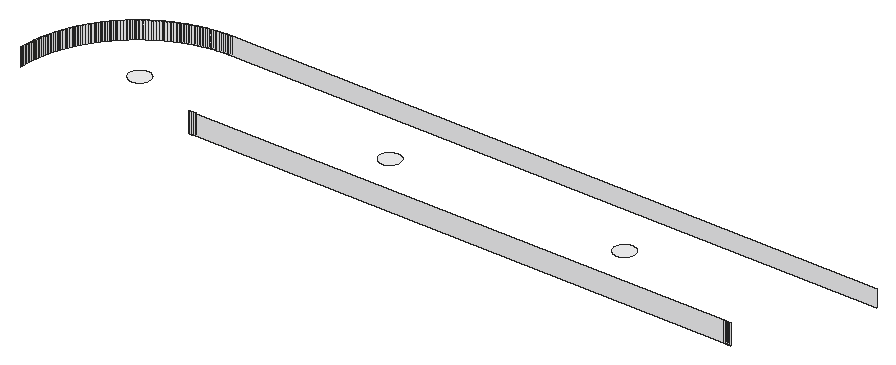
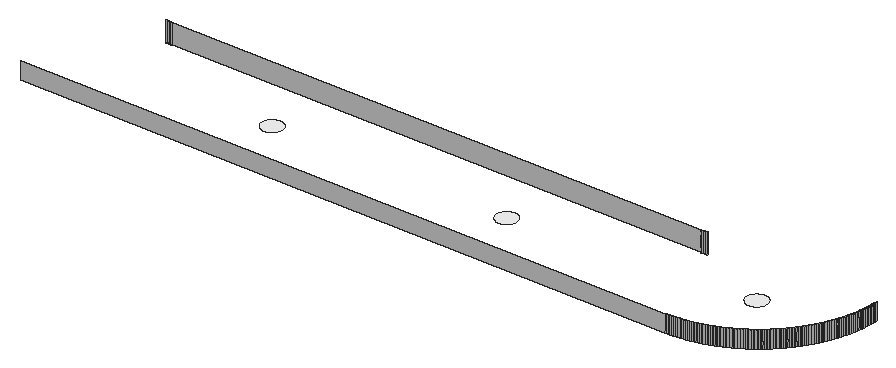
# SketchUp Ruby script. Lengths in inches.
U = 1.inch
M = Sketchup.active_model
def pt(a) = Geom::Point3d.new(a.map { |v| v * U })
def face(e, loops, mat)
  f = e.add_face(loops[0].map { |a| pt(a) })
  loops[1..].each { |l| e.add_face(l.map { |a| pt(a) }).erase! }
  f.material = f.back_material = mat if mat
  f
end
# faces: each face lists its corners as indices into pts; further lists are holes
def faces(e, pts, list, mat = nil) = list.each { |f| face(e, (f[0].is_a?(Array) ? f : [f]).map { |l| l.map { |i| pts[i] } }, mat) }
# xy, xz, yz: faces in a plane at the given z, y or x. An outline is a flat list of corners, or four numbers for a rectangle; further outlines are holes
def ring(l) = l.size == 4 ? [[l[0], l[1]], [l[2], l[1]], [l[2], l[3]], [l[0], l[3]]] : l.each_slice(2).to_a
def flat(e, list, mat, &to3) = list.each { |f| face(e, (f[0].is_a?(Array) ? f : [f]).map { |l| ring(l).map { |u, v| to3.(u, v) } }, mat) }
def xy(e, z, list, mat = nil) = flat(e, list, mat) { |x, y| [x, y, z] }
def xz(e, y, list, mat = nil) = flat(e, list, mat) { |x, z| [x, y, z] }
def yz(e, x, list, mat = nil) = flat(e, list, mat) { |y, z| [x, y, z] }
def lines(e, pts, list) = list.each { |a, b| e.add_line(pt(pts[a]), pt(pts[b])) }
# prism: a flat outline (further loops are holes) pulled along v
def prism(e, loops, v, mat = nil)
  f = face(e, loops, mat); d = Geom::Vector3d.new(v.map { |x| x * U })
  f.pushpull(f.normal.samedirection?(d) ? d.length : -d.length)
end
def box(e, o, s, mat = nil) = prism(e, [[o, [o[0] + s[0], o[1], o[2]], [o[0] + s[0], o[1] + s[1], o[2]], [o[0], o[1] + s[1], o[2]]]], [0, 0, s[2]], mat)
def at(x, y, z, deg = 0) = Geom::Transformation.translation(pt([x, y, z])) * Geom::Transformation.rotation(ORIGIN, Z_AXIS, deg.degrees)
def axes(o, x, y, z) = Geom::Transformation.new([*x, 0, *y, 0, *z, 0, *pt(o).to_a, 1])
def part(name) = M.definitions.add(name)
# library, detail: a bought-in or finely detailed component or shape, given as its bounding box
def library(name, o, s) = part(name).tap { |d| box(d.entities, o, s) }
def detail(e, o, s) = box(e.add_group.entities, o, s)
def put(e, d, t, mat = nil) = e.add_instance(d, t).tap { |i| i.material = mat if mat }
def group(e, t, mat = nil) = e.add_group.tap { |g| g.transformation = t; g.material = mat if mat }.entities
root = M.entities
M.materials.add("[Quartz Light Grey]").color = [251, 251, 252]
xy(root,112.81,[[38.9375,222.06,38.9,222.07,38.8125,222.07,38.77,222.08,38.73,222.08,38.6875,222.09,38.65,222.09,38.625,222.1,38.6,222.1,38.5625,222.11,38.52,222.12,38.4,222.15,38.36,222.17,38.32,222.18,38.28,222.2,38.26,222.2,38.24,222.21,38.21,222.23,38.17,222.24,38.09,222.28,38.06,222.3,38.04,222.3125,38.02,222.32,37.98,222.34,37.95,222.36,37.91,222.39,37.84,222.43,37.81,222.46,37.77,222.48,37.71,222.54,37.68,222.5625,37.65,222.59,37.56,222.68,37.54,222.69,37.53,222.71,37.47,222.77,37.46,222.79,37.45,222.8,37.42,222.84,37.39,222.87,37.38,222.89,37.37,222.9,37.35,222.9375,37.32,222.97,37.3125,222.99,37.3,223.01,37.28,223.05,37.26,223.08,37.22,223.16,37.2,223.19,37.18,223.23,37.17,223.27,37.13,223.35,37.12,223.39,37.1,223.42,37.1,223.44,37.09,223.47,37.08,223.51,37.07,223.54,37.0625,223.57,37.06,223.59,37.05,223.625,37.04,223.67,37.04,223.6875,37.03,223.71,37.03,223.75,37.02,223.79,37.02,223.8125,37.01,223.83,37.01,223.92,37,223.9375,37,224.1875,37.01,224.21,37.01,224.29,37.02,224.3125,37.02,224.33,37.03,224.375,37.03,224.42,37.04,224.4375,37.04,224.46,37.06,224.54,37.0625,224.56,37.07,224.58,37.09,224.66,37.1,224.68,37.1,224.7,37.12,224.74,37.13,224.78,37.17,224.86,37.18,224.89,37.26,225.05,37.28,225.08,37.3,225.12,37.3125,225.13,37.32,225.15,37.35,225.1875,37.37,225.22,37.39,225.26,37.45,225.32,37.46,225.34,37.5,225.38,37.53,225.42,37.65,225.54,37.68,225.5625,37.71,225.59,37.73,225.6,37.74,225.62,37.77,225.64,37.81,225.67,37.82,225.68,37.84,225.69,37.875,225.72,37.91,225.74,37.95,225.76,37.98,225.78,38.04,225.81,38.06,225.83,38.09,225.84,38.21,225.9,38.24,225.91,38.28,225.93,38.32,225.94,38.36,225.96,38.38,225.96,38.4,225.97,38.48,225.99,38.52,226.01,38.5625,226.01,38.6,226.02,38.625,226.03,38.65,226.03,38.6875,226.04,38.73,226.04,38.75,226.05,38.8125,226.05,38.85,226.06,38.9,226.06,38.9375,226.0625,39.0625,226.0625,39.1,226.06,39.15,226.06,39.1875,226.05,39.25,226.05,39.27,226.04,39.3125,226.04,39.35,226.03,39.375,226.03,39.4,226.02,39.4375,226.01,39.48,226.01,39.52,225.99,39.6,225.97,39.62,225.96,39.64,225.96,39.68,225.94,39.72,225.93,39.76,225.91,39.79,225.9,39.91,225.84,39.94,225.83,39.96,225.81,40.02,225.78,40.05,225.76,40.09,225.74,40.125,225.72,40.16,225.69,40.18,225.68,40.19,225.67,40.23,225.64,40.26,225.62,40.27,225.6,40.29,225.59,40.32,225.5625,40.35,225.54,40.47,225.42,40.5,225.38,40.54,225.34,40.55,225.32,40.61,225.26,40.63,225.22,40.65,225.1875,40.68,225.15,40.6875,225.13,40.7,225.12,40.72,225.08,40.74,225.05,40.82,224.89,40.83,224.86,40.87,224.78,40.88,224.74,40.9,224.7,40.9,224.68,40.91,224.66,40.93,224.58,40.9375,224.56,40.94,224.54,40.96,224.46,40.96,224.4375,40.97,224.42,40.97,224.375,40.98,224.33,40.98,224.3125,40.99,224.29,40.99,224.21,41,224.1875,41,223.9375,40.99,223.92,40.99,223.83,40.98,223.8125,40.98,223.79,40.97,223.75,40.97,223.71,40.96,223.6875,40.96,223.67,40.95,223.625,40.94,223.59,40.9375,223.57,40.93,223.54,40.92,223.51,40.91,223.47,40.9,223.44,40.9,223.42,40.88,223.39,40.87,223.35,40.83,223.27,40.82,223.23,40.8,223.19,40.78,223.16,40.74,223.08,40.72,223.05,40.7,223.01,40.6875,222.99,40.68,222.97,40.65,222.9375,40.63,222.9,40.62,222.89,40.61,222.87,40.58,222.84,40.55,222.8,40.54,222.79,40.53,222.77,40.47,222.71,40.46,222.69,40.44,222.68,40.35,222.59,40.32,222.5625,40.29,222.54,40.23,222.48,40.19,222.46,40.16,222.43,40.09,222.39,40.05,222.36,40.02,222.34,39.98,222.32,39.96,222.3125,39.94,222.3,39.91,222.28,39.83,222.24,39.79,222.23,39.76,222.21,39.74,222.2,39.72,222.2,39.68,222.18,39.64,222.17,39.6,222.15,39.48,222.12,39.4375,222.11,39.4,222.1,39.375,222.1,39.35,222.09,39.3125,222.09,39.27,222.08,39.23,222.08,39.1875,222.07,39.1,222.07,39.0625,222.06,39.02,222.0625,38.98,222.0625],[86.98,226.0625,86.85,226.07,86.73,226.08,86.6,226.1,86.48,226.13,86.24,226.21,86.13,226.26,86.02,226.32,85.91,226.39,85.81,226.46,85.71,226.54,85.62,226.62,85.53,226.71,85.45,226.8,85.37,226.9,85.3,227.01,85.18,227.23,85.13,227.35,85.09,227.47,85.03,227.71,85.01,227.83,85,227.96,85,228.08,85.01,228.21,85.02,228.33,85.04,228.46,85.1,228.7,85.15,228.82,85.2,228.93,85.26,229.05,85.32,229.15,85.39,229.26,85.47,229.35,85.56,229.45,85.65,229.54,85.74,229.62,85.84,229.69,86.06,229.83,86.28,229.93,86.52,230.01,86.65,230.03,86.77,230.05,86.9,230.06,87.02,230.0625,87.15,230.06,87.27,230.04,87.4,230.02,87.64,229.96,87.76,229.91,87.87,229.86,88.09,229.74,88.19,229.67,88.29,229.59,88.38,229.51,88.47,229.42,88.63,229.22,88.7,229.12,88.76,229.01,88.82,228.89,88.87,228.78,88.91,228.66,88.97,228.42,88.99,228.29,89,228.17,89,228.04,88.99,227.92,88.98,227.79,88.96,227.67,88.93,227.54,88.9,227.42,88.85,227.31,88.8,227.19,88.68,226.97,88.61,226.87,88.53,226.77,88.35,226.59,88.26,226.51,88.16,226.43,88.05,226.36,87.83,226.24,87.72,226.2,87.6,226.15,87.48,226.12,87.35,226.09,87.23,226.08,87.1,226.07],[134.98,226.0625,134.85,226.07,134.73,226.08,134.6,226.1,134.48,226.13,134.24,226.21,134.13,226.26,134.02,226.32,133.91,226.39,133.81,226.46,133.71,226.54,133.62,226.62,133.53,226.71,133.45,226.8,133.37,226.9,133.3,227.01,133.18,227.23,133.13,227.35,133.09,227.47,133.03,227.71,133.01,227.83,133,227.96,133,228.08,133.01,228.21,133.02,228.33,133.04,228.46,133.1,228.7,133.15,228.82,133.2,228.93,133.26,229.05,133.32,229.15,133.39,229.26,133.47,229.35,133.56,229.45,133.65,229.54,133.74,229.62,133.84,229.69,134.06,229.83,134.28,229.93,134.52,230.01,134.65,230.03,134.77,230.05,134.9,230.06,135.02,230.0625,135.15,230.06,135.27,230.04,135.4,230.02,135.64,229.96,135.76,229.91,135.87,229.86,136.09,229.74,136.19,229.67,136.29,229.59,136.38,229.51,136.47,229.42,136.63,229.22,136.7,229.12,136.76,229.01,136.82,228.89,136.87,228.78,136.91,228.66,136.97,228.42,136.99,228.29,137,228.17,137,228.04,136.99,227.92,136.98,227.79,136.96,227.67,136.93,227.54,136.9,227.42,136.85,227.31,136.8,227.19,136.68,226.97,136.61,226.87,136.53,226.77,136.35,226.59,136.26,226.51,136.16,226.43,136.05,226.36,135.83,226.24,135.72,226.2,135.6,226.15,135.48,226.12,135.35,226.09,135.23,226.08,135.1,226.07]],"[Quartz Light Grey]")
xz(root,216,[[56.6875,111.81,56.84,115.91],[56.84,111.81,57,115.91],[57,111.81,165,115.91],[165,111.81,165.16,115.91],[165.16,111.81,165.3125,115.91]],"[Quartz Light Grey]")
xz(root,239.99,[[44.25,111.81,44.5,115.32]],"[Quartz Light Grey]")
xz(root,240,[[44.75,111.81,45,115.32],[45,111.81,177,115.32]],"[Quartz Light Grey]")
yz(root,21,[[216,111.81,216.25,115.32]],"[Quartz Light Grey]")
yz(root,21.01,[[216.5,111.81,216.75,115.32]],"[Quartz Light Grey]")
p = [[55.59,215.92,111.81],[55.75,215.93,111.81],[55.75,215.93,115.91],[55.59,215.92,115.91],[55.9,215.95,111.81],[55.9,215.95,115.91],
  [56.06,215.96,111.81],[56.06,215.96,115.91],[165.94,215.96,111.81],[166.1,215.95,111.81],[166.1,215.95,115.91],[165.94,215.96,115.91],
  [166.25,215.93,111.81],[166.25,215.93,115.91],[166.41,215.92,111.81],[166.41,215.92,115.91],[56.22,215.97,111.81],[56.22,215.97,115.91],
  [56.37,215.98,111.81],[56.37,215.98,115.91],[56.53,215.99,111.81],[56.53,215.99,115.91],[56.6875,216,111.81],[56.6875,216,115.91],
  [165.3125,216,111.81],[165.47,215.99,111.81],[165.47,215.99,115.91],[165.3125,216,115.91],[165.63,215.98,111.81],[165.63,215.98,115.91],
  [165.78,215.97,111.81],[165.78,215.97,115.91],[21.01,216.5,111.81],[21,216.25,111.81],[21,216.25,115.32],[21.01,216.5,115.32],
  [21.02,217.01,111.81],[21.01,216.75,111.81],[21.01,216.75,115.32],[21.02,217.01,115.32],[21.03,217.26,111.81],[21.03,217.26,115.32],
  [21.05,217.51,111.81],[21.05,217.51,115.32],[21.0625,217.76,111.81],[21.0625,217.76,115.32],[21.08,218.01,111.81],[21.08,218.01,115.32],
  [21.11,218.26,111.81],[21.11,218.26,115.32],[21.13,218.51,111.81],[21.13,218.51,115.32],[21.16,218.76,111.81],[21.16,218.76,115.32],
  [21.1875,219.01,111.81],[21.1875,219.01,115.32],[21.22,219.26,111.81],[21.22,219.26,115.32],[21.26,219.51,111.81],[21.26,219.51,115.32],
  [21.3,219.75,111.81],[21.3,219.75,115.32],[21.34,220,111.81],[21.34,220,115.32],[21.38,220.25,111.81],[21.38,220.25,115.32],
  [21.43,220.5,111.81],[21.43,220.5,115.32],[21.47,220.74,111.81],[21.47,220.74,115.32],[21.52,220.99,111.81],[21.52,220.99,115.32],
  [21.58,221.24,111.81],[21.58,221.24,115.32],[21.63,221.48,111.81],[21.63,221.48,115.32],[21.69,221.72,111.81],[21.69,221.72,115.32],
  [21.75,221.97,111.81],[21.75,221.97,115.32],[21.82,222.21,111.81],[21.82,222.21,115.32],[21.88,222.45,111.81],[21.88,222.45,115.32],
  [21.95,222.7,111.81],[21.95,222.7,115.32],[22.02,222.9375,111.81],[22.02,222.9375,115.32],[22.1,223.18,111.81],[22.1,223.18,115.32],
  [22.17,223.42,111.81],[22.17,223.42,115.32],[22.25,223.66,111.81],[22.25,223.66,115.32],[22.33,223.89,111.81],[22.33,223.89,115.32],
  [22.42,224.13,111.81],[22.42,224.13,115.32],[22.51,224.37,111.81],[22.51,224.37,115.32],[22.59,224.6,111.81],[22.59,224.6,115.32],
  [22.69,224.83,111.81],[22.69,224.83,115.32],[22.78,225.07,111.81],[22.78,225.07,115.32],[22.875,225.3,111.81],[22.875,225.3,115.32],
  [22.97,225.53,111.81],[22.97,225.53,115.32],[23.07,225.76,111.81],[23.07,225.76,115.32],[23.18,225.99,111.81],[23.18,225.99,115.32],
  [23.28,226.22,111.81],[23.28,226.22,115.32],[23.39,226.45,111.81],[23.39,226.45,115.32],[23.5,226.67,111.81],[23.5,226.67,115.32],
  [23.62,226.9,111.81],[23.62,226.9,115.32],[23.73,227.12,111.81],[23.73,227.12,115.32],[23.85,227.34,111.81],[23.85,227.34,115.32],
  [23.97,227.5625,111.81],[23.97,227.5625,115.32],[24.09,227.78,111.81],[24.09,227.78,115.32],[24.22,228,111.81],[24.22,228,115.32],
  [24.34,228.22,111.81],[24.34,228.22,115.32],[24.47,228.43,111.81],[24.47,228.43,115.32],[24.6,228.65,111.81],[24.6,228.65,115.32],
  [24.74,228.86,111.81],[24.74,228.86,115.32],[24.87,229.07,111.81],[24.87,229.07,115.32],[25.01,229.28,111.81],[25.01,229.28,115.32],
  [25.15,229.49,111.81],[25.15,229.49,115.32],[25.29,229.7,111.81],[25.29,229.7,115.32],[25.4375,229.9,111.81],[25.4375,229.9,115.32],
  [25.58,230.11,111.81],[25.58,230.11,115.32],[25.73,230.31,111.81],[25.73,230.31,115.32],[25.88,230.51,111.81],[25.88,230.51,115.32],
  [26.04,230.71,111.81],[26.04,230.71,115.32],[26.19,230.91,111.81],[26.19,230.91,115.32],[26.35,231.1,111.81],[26.35,231.1,115.32],
  [26.51,231.3,111.81],[26.51,231.3,115.32],[26.67,231.49,111.81],[26.67,231.49,115.32],[26.83,231.68,111.81],[26.83,231.68,115.32],
  [27,231.87,111.81],[27,231.87,115.32],[27.16,232.06,111.81],[27.16,232.06,115.32],[27.33,232.25,111.81],[27.33,232.25,115.32],
  [27.5,232.43,111.81],[27.5,232.43,115.32],[27.68,232.61,111.81],[27.68,232.61,115.32],[27.85,232.79,111.81],[27.85,232.79,115.32],
  [28.03,232.97,111.81],[28.03,232.97,115.32],[28.21,233.15,111.81],[28.21,233.15,115.32],[28.39,233.32,111.81],[28.39,233.32,115.32],
  [28.57,233.5,111.81],[28.57,233.5,115.32],[28.75,233.67,111.81],[28.75,233.67,115.32],[28.94,233.84,111.81],[28.94,233.84,115.32],
  [29.13,234,111.81],[29.13,234,115.32],[29.32,234.17,111.81],[29.32,234.17,115.32],[29.51,234.33,111.81],[29.51,234.33,115.32],
  [29.7,234.49,111.81],[29.7,234.49,115.32],[29.9,234.65,111.81],[29.9,234.65,115.32],[30.09,234.81,111.81],[30.09,234.81,115.32],
  [30.29,234.96,111.81],[30.29,234.96,115.32],[30.49,235.12,111.81],[30.49,235.12,115.32],[30.69,235.27,111.81],[30.69,235.27,115.32],
  [30.89,235.42,111.81],[30.89,235.42,115.32],[31.1,235.5625,111.81],[31.1,235.5625,115.32],[31.3,235.71,111.81],[31.3,235.71,115.32],
  [31.51,235.85,111.81],[31.51,235.85,115.32],[31.72,235.99,111.81],[31.72,235.99,115.32],[31.93,236.13,111.81],[31.93,236.13,115.32],
  [32.14,236.26,111.81],[32.14,236.26,115.32],[32.35,236.4,111.81],[32.35,236.4,115.32],[32.57,236.53,111.81],[32.57,236.53,115.32],
  [32.78,236.66,111.81],[32.78,236.66,115.32],[33,236.78,111.81],[33,236.78,115.32],[33.22,236.91,111.81],[33.22,236.91,115.32],
  [33.4375,237.03,111.81],[33.4375,237.03,115.32],[33.66,237.15,111.81],[33.66,237.15,115.32],[33.88,237.27,111.81],[33.88,237.27,115.32],
  [34.1,237.38,111.81],[34.1,237.38,115.32],[34.33,237.5,111.81],[34.33,237.5,115.32],[34.55,237.61,111.81],[34.55,237.61,115.32],
  [34.78,237.72,111.81],[34.78,237.72,115.32],[35.01,237.82,111.81],[35.01,237.82,115.32],[35.24,237.93,111.81],[35.24,237.93,115.32],
  [35.47,238.03,111.81],[35.47,238.03,115.32],[35.7,238.125,111.81],[35.7,238.125,115.32],[35.93,238.22,111.81],[35.93,238.22,115.32],
  [36.17,238.31,111.81],[36.17,238.31,115.32],[36.4,238.41,111.81],[36.4,238.41,115.32],[36.63,238.49,111.81],[36.63,238.49,115.32],
  [36.87,238.58,111.81],[36.87,238.58,115.32],[37.11,238.67,111.81],[37.11,238.67,115.32],[37.34,238.75,111.81],[37.34,238.75,115.32],
  [37.58,238.83,111.81],[37.58,238.83,115.32],[37.82,238.9,111.81],[37.82,238.9,115.32],[38.0625,238.98,111.81],[38.0625,238.98,115.32],
  [38.3,239.05,111.81],[38.3,239.05,115.32],[38.55,239.12,111.81],[38.55,239.12,115.32],[38.79,239.18,111.81],[38.79,239.18,115.32],
  [39.03,239.25,111.81],[39.03,239.25,115.32],[39.28,239.31,111.81],[39.28,239.31,115.32],[39.52,239.37,111.81],[39.52,239.37,115.32],
  [39.76,239.42,111.81],[39.76,239.42,115.32],[40.01,239.48,111.81],[40.01,239.48,115.32],[40.26,239.53,111.81],[40.26,239.53,115.32],
  [40.5,239.57,111.81],[40.5,239.57,115.32],[40.75,239.62,111.81],[40.75,239.62,115.32],[41,239.66,111.81],[41,239.66,115.32],
  [41.25,239.7,111.81],[41.25,239.7,115.32],[41.49,239.74,111.81],[41.49,239.74,115.32],[41.74,239.78,111.81],[41.74,239.78,115.32],
  [41.99,239.8125,111.81],[41.99,239.8125,115.32],[42.24,239.84,111.81],[42.24,239.84,115.32],[42.49,239.87,111.81],[42.49,239.87,115.32],
  [42.74,239.89,111.81],[42.74,239.89,115.32],[42.99,239.92,111.81],[42.99,239.92,115.32],[43.24,239.9375,111.81],[43.24,239.9375,115.32],
  [43.49,239.95,111.81],[43.49,239.95,115.32],[43.74,239.97,111.81],[43.74,239.97,115.32],[43.99,239.98,111.81],[43.99,239.98,115.32],
  [44.25,239.99,111.81],[44.25,239.99,115.32],[44.75,240,111.81],[44.5,239.99,111.81],[44.5,239.99,115.32],[44.75,240,115.32]]
faces(root,p,[[0,1,2,3],[1,4,5,2],[4,6,7,5],[8,9,10,11],[9,12,13,10],[12,14,15,13],[6,16,17,7],[16,18,19,17],
  [18,20,21,19],[20,22,23,21],[24,25,26,27],[25,28,29,26],[28,30,31,29],[30,8,11,31],[32,33,34,35],[36,37,38,39],
  [40,36,39,41],[42,40,41,43],[44,42,43,45],[46,44,45,47],[48,46,47,49],[50,48,49,51],[52,50,51,53],[54,52,53,55],
  [56,54,55,57],[58,56,57,59],[60,58,59,61],[62,60,61,63],[64,62,63,65],[66,64,65,67],[68,66,67,69],[70,68,69,71],
  [72,70,71,73],[74,72,73,75],[76,74,75,77],[78,76,77,79],[80,78,79,81],[82,80,81,83],[84,82,83,85],[86,84,85,87],
  [88,86,87,89],[90,88,89,91],[92,90,91,93],[94,92,93,95],[96,94,95,97],[98,96,97,99],[100,98,99,101],[102,100,101,103],
  [104,102,103,105],[106,104,105,107],[108,106,107,109],[110,108,109,111],[112,110,111,113],[114,112,113,115],[116,114,115,117],[118,116,117,119],
  [120,118,119,121],[122,120,121,123],[124,122,123,125],[126,124,125,127],[128,126,127,129],[130,128,129,131],[132,130,131,133],[134,132,133,135],
  [136,134,135,137],[138,136,137,139],[140,138,139,141],[142,140,141,143],[144,142,143,145],[146,144,145,147],[148,146,147,149],[150,148,149,151],
  [152,150,151,153],[154,152,153,155],[156,154,155,157],[158,156,157,159],[160,158,159,161],[162,160,161,163],[164,162,163,165],[166,164,165,167],
  [168,166,167,169],[170,168,169,171],[172,170,171,173],[174,172,173,175],[176,174,175,177],[178,176,177,179],[180,178,179,181],[182,180,181,183],
  [184,182,183,185],[186,184,185,187],[188,186,187,189],[190,188,189,191],[192,190,191,193],[194,192,193,195],[196,194,195,197],[198,196,197,199],
  [200,198,199,201],[202,200,201,203],[204,202,203,205],[206,204,205,207],[208,206,207,209],[210,208,209,211],[212,210,211,213],[214,212,213,215],
  [216,214,215,217],[218,216,217,219],[220,218,219,221],[222,220,221,223],[224,222,223,225],[226,224,225,227],[228,226,227,229],[230,228,229,231],
  [232,230,231,233],[234,232,233,235],[236,234,235,237],[238,236,237,239],[240,238,239,241],[242,240,241,243],[244,242,243,245],[246,244,245,247],
  [248,246,247,249],[250,248,249,251],[252,250,251,253],[254,252,253,255],[256,254,255,257],[258,256,257,259],[260,258,259,261],[262,260,261,263],
  [264,262,263,265],[266,264,265,267],[268,266,267,269],[270,268,269,271],[272,270,271,273],[274,272,273,275],[276,274,275,277],[278,276,277,279],
  [280,278,279,281],[282,280,281,283],[284,282,283,285],[286,284,285,287],[288,286,287,289],[290,288,289,291],[292,290,291,293],[294,292,293,295],
  [296,294,295,297],[298,296,297,299],[300,298,299,301],[302,300,301,303],[304,302,303,305],[306,304,305,307],[308,306,307,309],[310,308,309,311],
  [312,310,311,313],[314,312,313,315],[316,314,315,317],[318,316,317,319],[320,318,319,321],[322,320,321,323],[324,322,323,325],[326,327,328,329]],"[Quartz Light Grey]")
